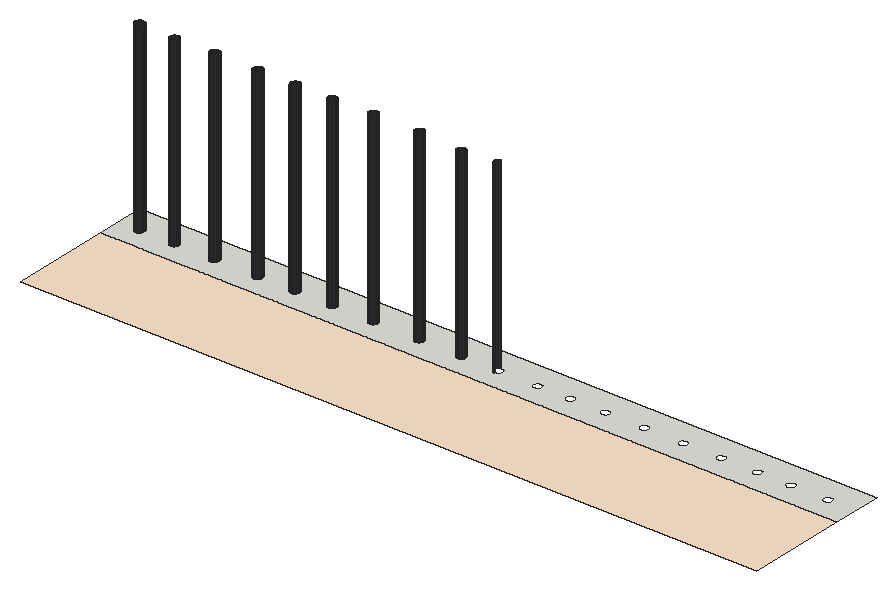
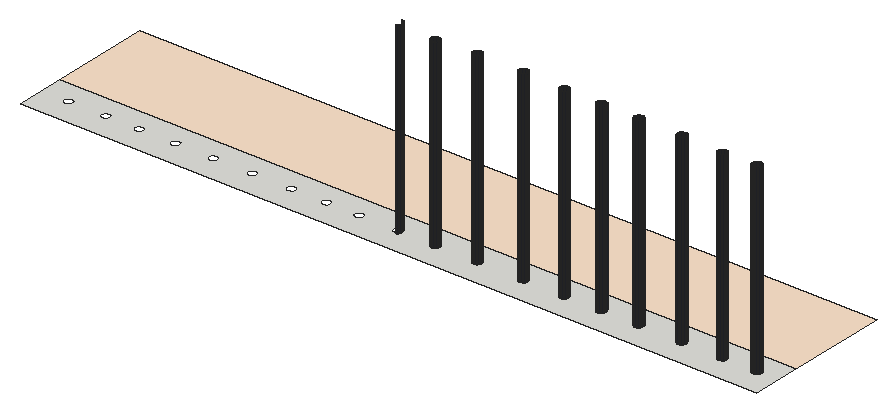
# SketchUp Ruby script. Lengths in inches.
U = 1.inch
M = Sketchup.active_model
def pt(a) = Geom::Point3d.new(a.map { |v| v * U })
def face(e, loops, mat)
  f = e.add_face(loops[0].map { |a| pt(a) })
  loops[1..].each { |l| e.add_face(l.map { |a| pt(a) }).erase! }
  f.material = f.back_material = mat if mat
  f
end
# faces: each face lists its corners as indices into pts; further lists are holes
def faces(e, pts, list, mat = nil) = list.each { |f| face(e, (f[0].is_a?(Array) ? f : [f]).map { |l| l.map { |i| pts[i] } }, mat) }
# xy, xz, yz: faces in a plane at the given z, y or x. An outline is a flat list of corners, or four numbers for a rectangle; further outlines are holes
def ring(l) = l.size == 4 ? [[l[0], l[1]], [l[2], l[1]], [l[2], l[3]], [l[0], l[3]]] : l.each_slice(2).to_a
def flat(e, list, mat, &to3) = list.each { |f| face(e, (f[0].is_a?(Array) ? f : [f]).map { |l| ring(l).map { |u, v| to3.(u, v) } }, mat) }
def xy(e, z, list, mat = nil) = flat(e, list, mat) { |x, y| [x, y, z] }
def xz(e, y, list, mat = nil) = flat(e, list, mat) { |x, z| [x, y, z] }
def yz(e, x, list, mat = nil) = flat(e, list, mat) { |y, z| [x, y, z] }
def lines(e, pts, list) = list.each { |a, b| e.add_line(pt(pts[a]), pt(pts[b])) }
# prism: a flat outline (further loops are holes) pulled along v
def prism(e, loops, v, mat = nil)
  f = face(e, loops, mat); d = Geom::Vector3d.new(v.map { |x| x * U })
  f.pushpull(f.normal.samedirection?(d) ? d.length : -d.length)
end
def box(e, o, s, mat = nil) = prism(e, [[o, [o[0] + s[0], o[1], o[2]], [o[0] + s[0], o[1] + s[1], o[2]], [o[0], o[1] + s[1], o[2]]]], [0, 0, s[2]], mat)
def at(x, y, z, deg = 0) = Geom::Transformation.translation(pt([x, y, z])) * Geom::Transformation.rotation(ORIGIN, Z_AXIS, deg.degrees)
def axes(o, x, y, z) = Geom::Transformation.new([*x, 0, *y, 0, *z, 0, *pt(o).to_a, 1])
def part(name) = M.definitions.add(name)
# library, detail: a bought-in or finely detailed component or shape, given as its bounding box
def library(name, o, s) = part(name).tap { |d| box(d.entities, o, s) }
def detail(e, o, s) = box(e.add_group.entities, o, s)
def put(e, d, t, mat = nil) = e.add_instance(d, t).tap { |i| i.material = mat if mat }
def group(e, t, mat = nil) = e.add_group.tap { |g| g.transformation = t; g.material = mat if mat }.entities
root = M.entities
M.materials.add("[Color C01]").color = [255, 229, 204]
M.materials.add("[Formica Laminate Dark]").color = [50, 53, 60]
xy(root,1179.9375,[[[746.18,769.97,1870.17,844.59],[1772.17,797.03,1770.375,797.27,1768.7,797.96,1767.27,799.06,1766.16,800.5,1765.47,802.17,1765.23,803.97,1765.47,805.77,1766.16,807.4375,1767.27,808.875,1768.7,809.98,1770.375,810.67,1772.17,810.91,1773.97,810.67,1775.64,809.98,1777.08,808.875,1778.18,807.4375,1778.87,805.77,1779.11,803.97,1778.87,802.17,1778.18,800.5,1777.08,799.06,1775.64,797.96,1773.97,797.27],[1205.55,797.03,1203.75,797.27,1202.08,797.96,1200.64,799.06,1199.54,800.5,1198.84,802.17,1198.61,803.97,1198.84,805.77,1199.54,807.4375,1200.64,808.875,1202.08,809.98,1203.75,810.67,1205.55,810.91,1207.34,810.67,1209.01,809.98,1210.45,808.875,1211.55,807.4375,1212.25,805.77,1212.48,803.97,1212.25,802.17,1211.55,800.5,1210.45,799.06,1209.01,797.96,1207.34,797.27],[1608.3,797.03,1606.5,797.27,1604.83,797.96,1603.39,799.06,1602.29,800.5,1601.59,802.17,1601.36,803.97,1601.59,805.77,1602.29,807.4375,1603.39,808.875,1604.83,809.98,1606.5,810.67,1608.3,810.91,1610.09,810.67,1611.76,809.98,1613.2,808.875,1614.3,807.4375,1615,805.77,1615.23,803.97,1615,802.17,1614.3,800.5,1613.2,799.06,1611.76,797.96,1610.09,797.27],[1326.55,797.03,1324.75,797.27,1323.08,797.96,1321.64,799.06,1320.54,800.5,1319.84,802.17,1319.61,803.97,1319.84,805.77,1320.54,807.4375,1321.64,808.875,1323.08,809.98,1324.75,810.67,1326.55,810.91,1328.34,810.67,1330.01,809.98,1331.45,808.875,1332.55,807.4375,1333.25,805.77,1333.48,803.97,1333.25,802.17,1332.55,800.5,1331.45,799.06,1330.01,797.96,1328.34,797.27],[1548.73,797.03,1546.9375,797.27,1545.26,797.96,1543.83,799.06,1542.73,800.5,1542.03,802.17,1541.8,803.97,1542.03,805.77,1542.73,807.4375,1543.83,808.875,1545.26,809.98,1546.9375,810.67,1548.73,810.91,1550.53,810.67,1552.2,809.98,1553.64,808.875,1554.74,807.4375,1555.43,805.77,1555.67,803.97,1555.43,802.17,1554.74,800.5,1553.64,799.06,1552.2,797.96,1550.53,797.27],[1435.55,797.03,1433.75,797.27,1432.08,797.96,1430.64,799.06,1429.54,800.5,1428.84,802.17,1428.61,803.97,1428.84,805.77,1429.54,807.4375,1430.64,808.875,1432.08,809.98,1433.75,810.67,1435.55,810.91,1437.34,810.67,1439.01,809.98,1440.45,808.875,1441.55,807.4375,1442.25,805.77,1442.48,803.97,1442.25,802.17,1441.55,800.5,1440.45,799.06,1439.01,797.96,1437.34,797.27],[1072.61,797.03,1070.8125,797.27,1069.14,797.96,1067.7,799.06,1066.6,800.5,1065.91,802.17,1065.67,803.97,1065.91,805.77,1066.6,807.4375,1067.7,808.875,1069.14,809.98,1070.8125,810.67,1072.61,810.91,1074.4,810.67,1076.08,809.98,1077.51,808.875,1078.62,807.4375,1079.31,805.77,1079.55,803.97,1079.31,802.17,1078.62,800.5,1077.51,799.06,1076.08,797.96,1074.4,797.27],[1721.48,797.03,1719.6875,797.27,1718.01,797.96,1716.58,799.06,1715.48,800.5,1714.78,802.17,1714.55,803.97,1714.78,805.77,1715.48,807.4375,1716.58,808.875,1718.01,809.98,1719.6875,810.67,1721.48,810.91,1723.28,810.67,1724.95,809.98,1726.39,808.875,1727.49,807.4375,1728.18,805.77,1728.42,803.97,1728.18,802.17,1727.49,800.5,1726.39,799.06,1724.95,797.96,1723.28,797.27],[778.8,797.03,777,797.27,775.33,797.96,773.89,799.06,772.79,800.5,772.09,802.17,771.86,803.97,772.09,805.77,772.79,807.4375,773.89,808.875,775.33,809.98,777,810.67,778.8,810.91,780.59,810.67,782.26,809.98,783.7,808.875,784.8,807.4375,785.5,805.77,785.73,803.97,785.5,802.17,784.8,800.5,783.7,799.06,782.26,797.96,780.59,797.27],[831.73,797.03,829.9375,797.27,828.26,797.96,826.83,799.06,825.73,800.5,825.03,802.17,824.8,803.97,825.03,805.77,825.73,807.4375,826.83,808.875,828.26,809.98,829.9375,810.67,831.73,810.91,833.53,810.67,835.2,809.98,836.64,808.875,837.74,807.4375,838.43,805.77,838.67,803.97,838.43,802.17,837.74,800.5,836.64,799.06,835.2,797.96,833.53,797.27],[893.3,797.03,891.5,797.27,889.83,797.96,888.39,799.06,887.29,800.5,886.59,802.17,886.36,803.97,886.59,805.77,887.29,807.4375,888.39,808.875,889.83,809.98,891.5,810.67,893.3,810.91,895.09,810.67,896.76,809.98,898.2,808.875,899.3,807.4375,900,805.77,900.23,803.97,900,802.17,899.3,800.5,898.2,799.06,896.76,797.96,895.09,797.27],[959.23,797.03,957.4375,797.27,955.76,797.96,954.33,799.06,953.23,800.5,952.53,802.17,952.3,803.97,952.53,805.77,953.23,807.4375,954.33,808.875,955.76,809.98,957.4375,810.67,959.23,810.91,961.03,810.67,962.7,809.98,964.14,808.875,965.24,807.4375,965.93,805.77,966.17,803.97,965.93,802.17,965.24,800.5,964.14,799.06,962.7,797.96,961.03,797.27],[1015.98,797.03,1014.1875,797.27,1012.51,797.96,1011.08,799.06,1009.98,800.5,1009.28,802.17,1009.05,803.97,1009.28,805.77,1009.98,807.4375,1011.08,808.875,1012.51,809.98,1014.1875,810.67,1015.98,810.91,1017.78,810.67,1019.45,809.98,1020.89,808.875,1021.99,807.4375,1022.68,805.77,1022.92,803.97,1022.68,802.17,1021.99,800.5,1020.89,799.06,1019.45,797.96,1017.78,797.27],[1135.17,797.03,1133.375,797.27,1131.7,797.96,1130.27,799.06,1129.16,800.5,1128.47,802.17,1128.23,803.97,1128.47,805.77,1129.16,807.4375,1130.27,808.875,1131.7,809.98,1133.375,810.67,1135.17,810.91,1136.97,810.67,1138.64,809.98,1140.08,808.875,1141.18,807.4375,1141.87,805.77,1142.11,803.97,1141.87,802.17,1141.18,800.5,1140.08,799.06,1138.64,797.96,1136.97,797.27],[1828.92,797.03,1827.125,797.27,1825.45,797.96,1824.02,799.06,1822.91,800.5,1822.22,802.17,1821.98,803.97,1822.22,805.77,1822.91,807.4375,1824.02,808.875,1825.45,809.98,1827.125,810.67,1828.92,810.91,1830.72,810.67,1832.39,809.98,1833.83,808.875,1834.93,807.4375,1835.62,805.77,1835.86,803.97,1835.62,802.17,1834.93,800.5,1833.83,799.06,1832.39,797.96,1830.72,797.27],[1665.86,797.03,1664.0625,797.27,1662.39,797.96,1660.95,799.06,1659.85,800.5,1659.16,802.17,1658.92,803.97,1659.16,805.77,1659.85,807.4375,1660.95,808.875,1662.39,809.98,1664.0625,810.67,1665.86,810.91,1667.65,810.67,1669.33,809.98,1670.76,808.875,1671.87,807.4375,1672.56,805.77,1672.8,803.97,1672.56,802.17,1671.87,800.5,1670.76,799.06,1669.33,797.96,1667.65,797.27],[1269.3,797.03,1267.5,797.27,1265.83,797.96,1264.39,799.06,1263.29,800.5,1262.59,802.17,1262.36,803.97,1262.59,805.77,1263.29,807.4375,1264.39,808.875,1265.83,809.98,1267.5,810.67,1269.3,810.91,1271.09,810.67,1272.76,809.98,1274.2,808.875,1275.3,807.4375,1276,805.77,1276.23,803.97,1276,802.17,1275.3,800.5,1274.2,799.06,1272.76,797.96,1271.09,797.27],[1386.05,797.03,1384.25,797.27,1382.58,797.96,1381.14,799.06,1380.04,800.5,1379.34,802.17,1379.11,803.97,1379.34,805.77,1380.04,807.4375,1381.14,808.875,1382.58,809.98,1384.25,810.67,1386.05,810.91,1387.84,810.67,1389.51,809.98,1390.95,808.875,1392.05,807.4375,1392.75,805.77,1392.98,803.97,1392.75,802.17,1392.05,800.5,1390.95,799.06,1389.51,797.96,1387.84,797.27],[1489.3,797.03,1487.5,797.27,1485.83,797.96,1484.39,799.06,1483.29,800.5,1482.59,802.17,1482.36,803.97,1482.59,805.77,1483.29,807.4375,1484.39,808.875,1485.83,809.98,1487.5,810.67,1489.3,810.91,1491.09,810.67,1492.76,809.98,1494.2,808.875,1495.3,807.4375,1496,805.77,1496.23,803.97,1496,802.17,1495.3,800.5,1494.2,799.06,1492.76,797.96,1491.09,797.27]],[778.8,797.03,777,797.27,775.33,797.96,773.89,799.06,772.79,800.5,772.09,802.17,771.86,803.97,772.09,805.77,772.79,807.4375,773.89,808.875,775.33,809.98,777,810.67,778.8,810.91,780.59,810.67,782.26,809.98,783.7,808.875,784.8,807.4375,785.5,805.77,785.73,803.97,785.5,802.17,784.8,800.5,783.7,799.06,782.26,797.96,780.59,797.27],[831.73,797.03,829.9375,797.27,828.26,797.96,826.83,799.06,825.73,800.5,825.03,802.17,824.8,803.97,825.03,805.77,825.73,807.4375,826.83,808.875,828.26,809.98,829.9375,810.67,831.73,810.91,833.53,810.67,835.2,809.98,836.64,808.875,837.74,807.4375,838.43,805.77,838.67,803.97,838.43,802.17,837.74,800.5,836.64,799.06,835.2,797.96,833.53,797.27],[893.3,797.03,891.5,797.27,889.83,797.96,888.39,799.06,887.29,800.5,886.59,802.17,886.36,803.97,886.59,805.77,887.29,807.4375,888.39,808.875,889.83,809.98,891.5,810.67,893.3,810.91,895.09,810.67,896.76,809.98,898.2,808.875,899.3,807.4375,900,805.77,900.23,803.97,900,802.17,899.3,800.5,898.2,799.06,896.76,797.96,895.09,797.27],[959.23,797.03,957.4375,797.27,955.76,797.96,954.33,799.06,953.23,800.5,952.53,802.17,952.3,803.97,952.53,805.77,953.23,807.4375,954.33,808.875,955.76,809.98,957.4375,810.67,959.23,810.91,961.03,810.67,962.7,809.98,964.14,808.875,965.24,807.4375,965.93,805.77,966.17,803.97,965.93,802.17,965.24,800.5,964.14,799.06,962.7,797.96,961.03,797.27],
  [1015.98,797.03,1014.1875,797.27,1012.51,797.96,1011.08,799.06,1009.98,800.5,1009.28,802.17,1009.05,803.97,1009.28,805.77,1009.98,807.4375,1011.08,808.875,1012.51,809.98,1014.1875,810.67,1015.98,810.91,1017.78,810.67,1019.45,809.98,1020.89,808.875,1021.99,807.4375,1022.68,805.77,1022.92,803.97,1022.68,802.17,1021.99,800.5,1020.89,799.06,1019.45,797.96,1017.78,797.27],[1072.61,797.03,1070.8125,797.27,1069.14,797.96,1067.7,799.06,1066.6,800.5,1065.91,802.17,1065.67,803.97,1065.91,805.77,1066.6,807.4375,1067.7,808.875,1069.14,809.98,1070.8125,810.67,1072.61,810.91,1074.4,810.67,1076.08,809.98,1077.51,808.875,1078.62,807.4375,1079.31,805.77,1079.55,803.97,1079.31,802.17,1078.62,800.5,1077.51,799.06,1076.08,797.96,1074.4,797.27],[1135.17,797.03,1133.375,797.27,1131.7,797.96,1130.27,799.06,1129.16,800.5,1128.47,802.17,1128.23,803.97,1128.47,805.77,1129.16,807.4375,1130.27,808.875,1131.7,809.98,1133.375,810.67,1135.17,810.91,1136.97,810.67,1138.64,809.98,1140.08,808.875,1141.18,807.4375,1141.87,805.77,1142.11,803.97,1141.87,802.17,1141.18,800.5,1140.08,799.06,1138.64,797.96,1136.97,797.27],[1205.55,797.03,1203.75,797.27,1202.08,797.96,1200.64,799.06,1199.54,800.5,1198.84,802.17,1198.61,803.97,1198.84,805.77,1199.54,807.4375,1200.64,808.875,1202.08,809.98,1203.75,810.67,1205.55,810.91,1207.34,810.67,1209.01,809.98,1210.45,808.875,1211.55,807.4375,1212.25,805.77,1212.48,803.97,1212.25,802.17,1211.55,800.5,1210.45,799.06,1209.01,797.96,1207.34,797.27],[1269.3,797.03,1267.5,797.27,1265.83,797.96,1264.39,799.06,1263.29,800.5,1262.59,802.17,1262.36,803.97,1262.59,805.77,1263.29,807.4375,1264.39,808.875,1265.83,809.98,1267.5,810.67,1269.3,810.91,1271.09,810.67,1272.76,809.98,1274.2,808.875,1275.3,807.4375,1276,805.77,1276.23,803.97,1276,802.17,1275.3,800.5,1274.2,799.06,1272.76,797.96,1271.09,797.27]])
xy(root,1179.9375,[[746.18,617.28,1870.17,769.97]],"[Color C01]")
p = [[777,797.27,1179.9375],[778.8,797.03,1179.9375],[778.8,797.03,1462.7],[777,797.27,1462.7],[780.59,797.27,1179.9375],[780.59,797.27,1462.7],
  [829.9375,797.27,1179.9375],[831.73,797.03,1179.9375],[831.73,797.03,1460.71],[829.9375,797.27,1460.71],[833.53,797.27,1179.9375],[833.53,797.27,1460.71],
  [891.5,797.27,1179.9375],[893.3,797.03,1179.9375],[893.3,797.03,1462.7],[891.5,797.27,1462.7],[895.09,797.27,1179.9375],[895.09,797.27,1462.7],
  [957.4375,797.27,1179.9375],[959.23,797.03,1179.9375],[959.23,797.03,1462.7],[957.4375,797.27,1462.7],[961.03,797.27,1179.9375],[961.03,797.27,1462.7],
  [1014.1875,797.27,1179.9375],[1015.98,797.03,1179.9375],[1015.98,797.03,1462.7],[1014.1875,797.27,1462.7],[1017.78,797.27,1179.9375],[1017.78,797.27,1462.7],
  [1070.8125,797.27,1179.9375],[1072.61,797.03,1179.9375],[1072.61,797.03,1462.7],[1070.8125,797.27,1462.7],[1074.4,797.27,1179.9375],[1074.4,797.27,1462.7],
  [1133.375,797.27,1179.9375],[1135.17,797.03,1179.9375],[1135.17,797.03,1464.6875],[1133.375,797.27,1464.6875],[1136.97,797.27,1179.9375],[1136.97,797.27,1464.6875],
  [1203.75,797.27,1179.9375],[1205.55,797.03,1179.9375],[1205.55,797.03,1464.6875],[1203.75,797.27,1464.6875],[1207.34,797.27,1179.9375],[1207.34,797.27,1464.6875],
  [1267.5,797.27,1179.9375],[1269.3,797.03,1179.9375],[1269.3,797.03,1460.9375],[1267.5,797.27,1460.9375],[1271.09,797.27,1179.9375],[1271.09,797.27,1460.9375],
  [1324.75,797.27,1179.9375],[1326.55,797.03,1179.9375],[1326.55,797.03,1464.6875],[1324.75,797.27,1464.6875],[775.33,797.96,1179.9375],[775.33,797.96,1462.7],
  [782.26,797.96,1179.9375],[782.26,797.96,1462.7],[828.26,797.96,1179.9375],[828.26,797.96,1460.71],[835.2,797.96,1179.9375],[835.2,797.96,1460.71],
  [889.83,797.96,1179.9375],[889.83,797.96,1462.7],[896.76,797.96,1179.9375],[896.76,797.96,1462.7],[955.76,797.96,1179.9375],[955.76,797.96,1462.7],
  [962.7,797.96,1179.9375],[962.7,797.96,1462.7],[1012.51,797.96,1179.9375],[1012.51,797.96,1462.7],[1019.45,797.96,1179.9375],[1019.45,797.96,1462.7],
  [1069.14,797.96,1179.9375],[1069.14,797.96,1462.7],[1076.08,797.96,1179.9375],[1076.08,797.96,1462.7],[1131.7,797.96,1179.9375],[1131.7,797.96,1464.6875],
  [1138.64,797.96,1179.9375],[1138.64,797.96,1464.6875],[1202.08,797.96,1179.9375],[1202.08,797.96,1464.6875],[1209.01,797.96,1179.9375],[1209.01,797.96,1464.6875],
  [1265.83,797.96,1179.9375],[1265.83,797.96,1460.9375],[1272.76,797.96,1179.9375],[1272.76,797.96,1460.9375],[1323.08,797.96,1179.9375],[1323.08,797.96,1464.6875],
  [773.89,799.06,1179.9375],[773.89,799.06,1462.7],[783.7,799.06,1179.9375],[783.7,799.06,1462.7],[826.83,799.06,1179.9375],[826.83,799.06,1460.71],
  [836.64,799.06,1179.9375],[836.64,799.06,1460.71],[888.39,799.06,1179.9375],[888.39,799.06,1462.7],[898.2,799.06,1179.9375],[898.2,799.06,1462.7],
  [954.33,799.06,1179.9375],[954.33,799.06,1462.7],[964.14,799.06,1179.9375],[964.14,799.06,1462.7],[1011.08,799.06,1179.9375],[1011.08,799.06,1462.7],
  [1020.89,799.06,1179.9375],[1020.89,799.06,1462.7],[1067.7,799.06,1179.9375],[1067.7,799.06,1462.7],[1077.51,799.06,1179.9375],[1077.51,799.06,1462.7],
  [1130.27,799.06,1179.9375],[1130.27,799.06,1464.6875],[1140.08,799.06,1179.9375],[1140.08,799.06,1464.6875],[1200.64,799.06,1179.9375],[1200.64,799.06,1464.6875],
  [1210.45,799.06,1179.9375],[1210.45,799.06,1464.6875],[1264.39,799.06,1179.9375],[1264.39,799.06,1460.9375],[1274.2,799.06,1179.9375],[1274.2,799.06,1460.9375],
  [1321.64,799.06,1179.9375],[1321.64,799.06,1464.6875],[772.79,800.5,1179.9375],[772.79,800.5,1462.7],[784.8,800.5,1179.9375],[784.8,800.5,1462.7],
  [825.73,800.5,1179.9375],[825.73,800.5,1460.71],[837.74,800.5,1179.9375],[837.74,800.5,1460.71],[887.29,800.5,1179.9375],[887.29,800.5,1462.7],
  [899.3,800.5,1179.9375],[899.3,800.5,1462.7],[953.23,800.5,1179.9375],[953.23,800.5,1462.7],[965.24,800.5,1179.9375],[965.24,800.5,1462.7],
  [1009.98,800.5,1179.9375],[1009.98,800.5,1462.7],[1021.99,800.5,1179.9375],[1021.99,800.5,1462.7],[1066.6,800.5,1179.9375],[1066.6,800.5,1462.7],
  [1078.62,800.5,1179.9375],[1078.62,800.5,1462.7],[1129.16,800.5,1179.9375],[1129.16,800.5,1464.6875],[1141.18,800.5,1179.9375],[1141.18,800.5,1464.6875],
  [1199.54,800.5,1179.9375],[1199.54,800.5,1464.6875],[1211.55,800.5,1179.9375],[1211.55,800.5,1464.6875],[1263.29,800.5,1179.9375],[1263.29,800.5,1460.9375],
  [1275.3,800.5,1179.9375],[1275.3,800.5,1460.9375],[1320.54,800.5,1179.9375],[1320.54,800.5,1464.6875],[772.09,802.17,1179.9375],[772.09,802.17,1462.7],
  [785.5,802.17,1179.9375],[785.5,802.17,1462.7],[825.03,802.17,1179.9375],[825.03,802.17,1460.71],[838.43,802.17,1179.9375],[838.43,802.17,1460.71],
  [886.59,802.17,1179.9375],[886.59,802.17,1462.7],[900,802.17,1179.9375],[900,802.17,1462.7],[952.53,802.17,1179.9375],[952.53,802.17,1462.7],
  [965.93,802.17,1179.9375],[965.93,802.17,1462.7],[1009.28,802.17,1179.9375],[1009.28,802.17,1462.7],[1022.68,802.17,1179.9375],[1022.68,802.17,1462.7],
  [1065.91,802.17,1179.9375],[1065.91,802.17,1462.7],[1079.31,802.17,1179.9375],[1079.31,802.17,1462.7],[1128.47,802.17,1179.9375],[1128.47,802.17,1464.6875],
  [1141.87,802.17,1179.9375],[1141.87,802.17,1464.6875],[1198.84,802.17,1179.9375],[1198.84,802.17,1464.6875],[1212.25,802.17,1179.9375],[1212.25,802.17,1464.6875],
  [1262.59,802.17,1179.9375],[1262.59,802.17,1460.9375],[1276,802.17,1179.9375],[1276,802.17,1460.9375],[1319.84,802.17,1179.9375],[1319.84,802.17,1464.6875],
  [771.86,803.97,1179.9375],[771.86,803.97,1462.7],[785.73,803.97,1179.9375],[785.73,803.97,1462.7],[824.8,803.97,1179.9375],[824.8,803.97,1460.71],
  [838.67,803.97,1179.9375],[838.67,803.97,1460.71],[886.36,803.97,1179.9375],[886.36,803.97,1462.7],[900.23,803.97,1179.9375],[900.23,803.97,1462.7],
  [952.3,803.97,1179.9375],[952.3,803.97,1462.7],[966.17,803.97,1179.9375],[966.17,803.97,1462.7],[1009.05,803.97,1179.9375],[1009.05,803.97,1462.7],
  [1022.92,803.97,1179.9375],[1022.92,803.97,1462.7],[1065.67,803.97,1179.9375],[1065.67,803.97,1462.7],[1079.55,803.97,1179.9375],[1079.55,803.97,1462.7],
  [1128.23,803.97,1179.9375],[1128.23,803.97,1464.6875],[1142.11,803.97,1179.9375],[1142.11,803.97,1464.6875],[1198.61,803.97,1179.9375],[1198.61,803.97,1464.6875],
  [1212.48,803.97,1179.9375],[1212.48,803.97,1464.6875],[1262.36,803.97,1179.9375],[1262.36,803.97,1460.9375],[1276.23,803.97,1179.9375],[1276.23,803.97,1460.9375],
  [1319.61,803.97,1179.9375],[1319.61,803.97,1464.6875],[772.09,805.77,1179.9375],[772.09,805.77,1462.7],[785.5,805.77,1179.9375],[785.5,805.77,1462.7],
  [825.03,805.77,1179.9375],[825.03,805.77,1460.71],[838.43,805.77,1179.9375],[838.43,805.77,1460.71],[886.59,805.77,1179.9375],[886.59,805.77,1462.7],
  [900,805.77,1179.9375],[900,805.77,1462.7],[952.53,805.77,1179.9375],[952.53,805.77,1462.7],[965.93,805.77,1179.9375],[965.93,805.77,1462.7],
  [1009.28,805.77,1179.9375],[1009.28,805.77,1462.7],[1022.68,805.77,1179.9375],[1022.68,805.77,1462.7],[1065.91,805.77,1179.9375],[1065.91,805.77,1462.7],
  [1079.31,805.77,1179.9375],[1079.31,805.77,1462.7],[1128.47,805.77,1179.9375],[1128.47,805.77,1464.6875],[1141.87,805.77,1179.9375],[1141.87,805.77,1464.6875],
  [1198.84,805.77,1179.9375],[1198.84,805.77,1464.6875],[1212.25,805.77,1179.9375],[1212.25,805.77,1464.6875],[1262.59,805.77,1179.9375],[1262.59,805.77,1460.9375],
  [1276,805.77,1179.9375],[1276,805.77,1460.9375],[1319.84,805.77,1179.9375],[1319.84,805.77,1464.6875],[772.79,807.4375,1179.9375],[772.79,807.4375,1462.7],
  [784.8,807.4375,1179.9375],[784.8,807.4375,1462.7],[825.73,807.4375,1179.9375],[825.73,807.4375,1460.71],[837.74,807.4375,1179.9375],[837.74,807.4375,1460.71],
  [887.29,807.4375,1179.9375],[887.29,807.4375,1462.7],[899.3,807.4375,1179.9375],[899.3,807.4375,1462.7],[953.23,807.4375,1179.9375],[953.23,807.4375,1462.7],
  [965.24,807.4375,1179.9375],[965.24,807.4375,1462.7],[1009.98,807.4375,1179.9375],[1009.98,807.4375,1462.7],[1021.99,807.4375,1179.9375],[1021.99,807.4375,1462.7],
  [1066.6,807.4375,1179.9375],[1066.6,807.4375,1462.7],[1078.62,807.4375,1179.9375],[1078.62,807.4375,1462.7],[1129.16,807.4375,1179.9375],[1129.16,807.4375,1464.6875],
  [1141.18,807.4375,1179.9375],[1141.18,807.4375,1464.6875],[1199.54,807.4375,1179.9375],[1199.54,807.4375,1464.6875],[1211.55,807.4375,1179.9375],[1211.55,807.4375,1464.6875],
  [1263.29,807.4375,1179.9375],[1263.29,807.4375,1460.9375],[1275.3,807.4375,1179.9375],[1275.3,807.4375,1460.9375],[1320.54,807.4375,1179.9375],[1320.54,807.4375,1464.6875],
  [773.89,808.875,1179.9375],[773.89,808.875,1462.7],[783.7,808.875,1179.9375],[783.7,808.875,1462.7],[826.83,808.875,1179.9375],[826.83,808.875,1460.71],
  [836.64,808.875,1179.9375],[836.64,808.875,1460.71],[888.39,808.875,1179.9375],[888.39,808.875,1462.7],[898.2,808.875,1179.9375],[898.2,808.875,1462.7],
  [954.33,808.875,1179.9375],[954.33,808.875,1462.7],[964.14,808.875,1179.9375],[964.14,808.875,1462.7],[1011.08,808.875,1179.9375],[1011.08,808.875,1462.7],
  [1020.89,808.875,1179.9375],[1020.89,808.875,1462.7],[1067.7,808.875,1179.9375],[1067.7,808.875,1462.7],[1077.51,808.875,1179.9375],[1077.51,808.875,1462.7],
  [1130.27,808.875,1179.9375],[1130.27,808.875,1464.6875],[1140.08,808.875,1179.9375],[1140.08,808.875,1464.6875],[1200.64,808.875,1179.9375],[1200.64,808.875,1464.6875],
  [1210.45,808.875,1179.9375],[1210.45,808.875,1464.6875],[1264.39,808.875,1179.9375],[1264.39,808.875,1460.9375],[1274.2,808.875,1179.9375],[1274.2,808.875,1460.9375],
  [1321.64,808.875,1179.9375],[1321.64,808.875,1464.6875],[775.33,809.98,1179.9375],[775.33,809.98,1462.7],[782.26,809.98,1179.9375],[782.26,809.98,1462.7],
  [828.26,809.98,1179.9375],[828.26,809.98,1460.71],[835.2,809.98,1179.9375],[835.2,809.98,1460.71],[889.83,809.98,1179.9375],[889.83,809.98,1462.7],
  [896.76,809.98,1179.9375],[896.76,809.98,1462.7],[955.76,809.98,1179.9375],[955.76,809.98,1462.7],[962.7,809.98,1179.9375],[962.7,809.98,1462.7],
  [1012.51,809.98,1179.9375],[1012.51,809.98,1462.7],[1019.45,809.98,1179.9375],[1019.45,809.98,1462.7],[1069.14,809.98,1179.9375],[1069.14,809.98,1462.7],
  [1076.08,809.98,1179.9375],[1076.08,809.98,1462.7],[1131.7,809.98,1179.9375],[1131.7,809.98,1464.6875],[1138.64,809.98,1179.9375],[1138.64,809.98,1464.6875],
  [1202.08,809.98,1179.9375],[1202.08,809.98,1464.6875],[1209.01,809.98,1179.9375],[1209.01,809.98,1464.6875],[1265.83,809.98,1179.9375],[1265.83,809.98,1460.9375],
  [1272.76,809.98,1179.9375],[1272.76,809.98,1460.9375],[1323.08,809.98,1179.9375],[1323.08,809.98,1464.6875],[777,810.67,1179.9375],[777,810.67,1462.7],
  [780.59,810.67,1179.9375],[780.59,810.67,1462.7],[829.9375,810.67,1179.9375],[829.9375,810.67,1460.71],[833.53,810.67,1179.9375],[833.53,810.67,1460.71],
  [891.5,810.67,1179.9375],[891.5,810.67,1462.7],[895.09,810.67,1179.9375],[895.09,810.67,1462.7],[957.4375,810.67,1179.9375],[957.4375,810.67,1462.7],
  [961.03,810.67,1179.9375],[961.03,810.67,1462.7],[1014.1875,810.67,1179.9375],[1014.1875,810.67,1462.7],[1017.78,810.67,1179.9375],[1017.78,810.67,1462.7],
  [1070.8125,810.67,1179.9375],[1070.8125,810.67,1462.7],[1074.4,810.67,1179.9375],[1074.4,810.67,1462.7],[1133.375,810.67,1179.9375],[1133.375,810.67,1464.6875],
  [1136.97,810.67,1179.9375],[1136.97,810.67,1464.6875],[1203.75,810.67,1179.9375],[1203.75,810.67,1464.6875],[1207.34,810.67,1179.9375],[1207.34,810.67,1464.6875],
  [1267.5,810.67,1179.9375],[1267.5,810.67,1460.9375],[1271.09,810.67,1179.9375],[1271.09,810.67,1460.9375],[1324.75,810.67,1179.9375],[1324.75,810.67,1464.6875],
  [778.8,810.91,1179.9375],[778.8,810.91,1462.7],[831.73,810.91,1179.9375],[831.05,810.82,1460.71],[831.73,810.91,1460.71],[832.41,810.82,1460.71],
  [893.3,810.91,1179.9375],[893.3,810.91,1462.7],[959.23,810.91,1179.9375],[959.23,810.91,1462.7],[1015.98,810.91,1179.9375],[1015.98,810.91,1462.7],
  [1072.61,810.91,1179.9375],[1072.61,810.91,1462.7],[1135.17,810.91,1179.9375],[1134.49,810.82,1464.6875],[1135.17,810.91,1464.6875],[1135.85,810.82,1464.6875],
  [1205.55,810.91,1179.9375],[1204.87,810.82,1464.6875],[1205.55,810.91,1464.6875],[1206.23,810.82,1464.6875],[1269.3,810.91,1179.9375],[1269.3,810.91,1460.9375]]
faces(root,p,[[0,1,2,3],[1,4,5,2],[6,7,8,9],[7,10,11,8],[12,13,14,15],[13,16,17,14],[18,19,20,21],[19,22,23,20],
  [24,25,26,27],[25,28,29,26],[30,31,32,33],[31,34,35,32],[36,37,38,39],[37,40,41,38],[42,43,44,45],[43,46,47,44],
  [48,49,50,51],[49,52,53,50],[54,55,56,57],[58,0,3,59],[4,60,61,5],[62,6,9,63],[10,64,65,11],[66,12,15,67],
  [16,68,69,17],[70,18,21,71],[22,72,73,23],[74,24,27,75],[28,76,77,29],[78,30,33,79],[34,80,81,35],[82,36,39,83],
  [40,84,85,41],[86,42,45,87],[46,88,89,47],[90,48,51,91],[52,92,93,53],[94,54,57,95],[96,58,59,97],[60,98,99,61],
  [100,62,63,101],[64,102,103,65],[104,66,67,105],[68,106,107,69],[108,70,71,109],[72,110,111,73],[112,74,75,113],[76,114,115,77],
  [116,78,79,117],[80,118,119,81],[120,82,83,121],[84,122,123,85],[124,86,87,125],[88,126,127,89],[128,90,91,129],[92,130,131,93],
  [132,94,95,133],[134,96,97,135],[98,136,137,99],[138,100,101,139],[102,140,141,103],[142,104,105,143],[106,144,145,107],[146,108,109,147],
  [110,148,149,111],[150,112,113,151],[114,152,153,115],[154,116,117,155],[118,156,157,119],[158,120,121,159],[122,160,161,123],[162,124,125,163],
  [126,164,165,127],[166,128,129,167],[130,168,169,131],[170,132,133,171],[172,134,135,173],[136,174,175,137],[176,138,139,177],[140,178,179,141],
  [180,142,143,181],[144,182,183,145],[184,146,147,185],[148,186,187,149],[188,150,151,189],[152,190,191,153],[192,154,155,193],[156,194,195,157],
  [196,158,159,197],[160,198,199,161],[200,162,163,201],[164,202,203,165],[204,166,167,205],[168,206,207,169],[208,170,171,209],[210,172,173,211],
  [174,212,213,175],[214,176,177,215],[178,216,217,179],[218,180,181,219],[182,220,221,183],[222,184,185,223],[186,224,225,187],[226,188,189,227],
  [190,228,229,191],[230,192,193,231],[194,232,233,195],[234,196,197,235],[198,236,237,199],[238,200,201,239],[202,240,241,203],[242,204,205,243],
  [206,244,245,207],[246,208,209,247],[248,210,211,249],[212,250,251,213],[252,214,215,253],[216,254,255,217],[256,218,219,257],[220,258,259,221],
  [260,222,223,261],[224,262,263,225],[264,226,227,265],[228,266,267,229],[268,230,231,269],[232,270,271,233],[272,234,235,273],[236,274,275,237],
  [276,238,239,277],[240,278,279,241],[280,242,243,281],[244,282,283,245],[284,246,247,285],[286,248,249,287],[250,288,289,251],[290,252,253,291],
  [254,292,293,255],[294,256,257,295],[258,296,297,259],[298,260,261,299],[262,300,301,263],[302,264,265,303],[266,304,305,267],[306,268,269,307],
  [270,308,309,271],[310,272,273,311],[274,312,313,275],[314,276,277,315],[278,316,317,279],[318,280,281,319],[282,320,321,283],[322,284,285,323],
  [324,286,287,325],[288,326,327,289],[328,290,291,329],[292,330,331,293],[332,294,295,333],[296,334,335,297],[336,298,299,337],[300,338,339,301],
  [340,302,303,341],[304,342,343,305],[344,306,307,345],[308,346,347,309],[348,310,311,349],[312,350,351,313],[352,314,315,353],[316,354,355,317],
  [356,318,319,357],[320,358,359,321],[360,322,323,361],[362,324,325,363],[326,364,365,327],[366,328,329,367],[330,368,369,331],[370,332,333,371],
  [334,372,373,335],[374,336,337,375],[338,376,377,339],[378,340,341,379],[342,380,381,343],[382,344,345,383],[346,384,385,347],[386,348,349,387],
  [350,388,389,351],[390,352,353,391],[354,392,393,355],[394,356,357,395],[358,396,397,359],[398,360,361,399],[400,362,363,401],[364,402,403,365],
  [404,366,367,405],[368,406,407,369],[408,370,371,409],[372,410,411,373],[412,374,375,413],[376,414,415,377],[416,378,379,417],[380,418,419,381],
  [420,382,383,421],[384,422,423,385],[424,386,387,425],[388,426,427,389],[428,390,391,429],[392,430,431,393],[432,394,395,433],[396,434,435,397],
  [436,398,399,437],[438,400,401,439],[402,438,439,403],[440,404,405,441,442],[406,440,442,443,407],[444,408,409,445],[410,444,445,411],[446,412,413,447],
  [414,446,447,415],[448,416,417,449],[418,448,449,419],[450,420,421,451],[422,450,451,423],[452,424,425,453,454],[426,452,454,455,427],[456,428,429,457,458],
  [430,456,458,459,431],[460,432,433,461],[434,460,461,435]],"[Formica Laminate Dark]")
